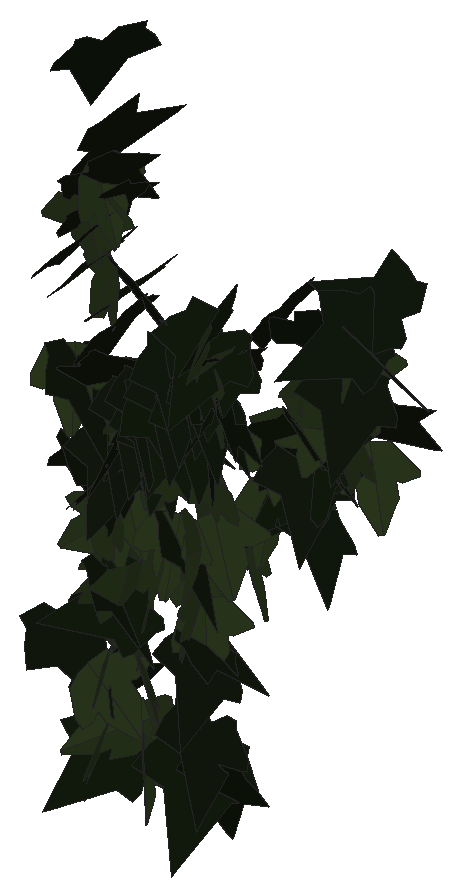
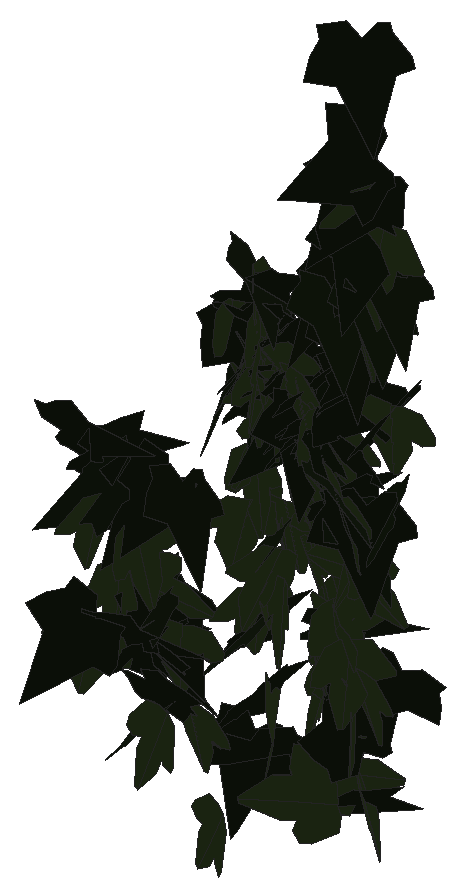
# SketchUp Ruby script. Lengths in inches.
U = 1.inch
M = Sketchup.active_model
def pt(a) = Geom::Point3d.new(a.map { |v| v * U })
def face(e, loops, mat)
  f = e.add_face(loops[0].map { |a| pt(a) })
  loops[1..].each { |l| e.add_face(l.map { |a| pt(a) }).erase! }
  f.material = f.back_material = mat if mat
  f
end
# faces: each face lists its corners as indices into pts; further lists are holes
def faces(e, pts, list, mat = nil) = list.each { |f| face(e, (f[0].is_a?(Array) ? f : [f]).map { |l| l.map { |i| pts[i] } }, mat) }
# xy, xz, yz: faces in a plane at the given z, y or x. An outline is a flat list of corners, or four numbers for a rectangle; further outlines are holes
def ring(l) = l.size == 4 ? [[l[0], l[1]], [l[2], l[1]], [l[2], l[3]], [l[0], l[3]]] : l.each_slice(2).to_a
def flat(e, list, mat, &to3) = list.each { |f| face(e, (f[0].is_a?(Array) ? f : [f]).map { |l| ring(l).map { |u, v| to3.(u, v) } }, mat) }
def xy(e, z, list, mat = nil) = flat(e, list, mat) { |x, y| [x, y, z] }
def xz(e, y, list, mat = nil) = flat(e, list, mat) { |x, z| [x, y, z] }
def yz(e, x, list, mat = nil) = flat(e, list, mat) { |y, z| [x, y, z] }
def lines(e, pts, list) = list.each { |a, b| e.add_line(pt(pts[a]), pt(pts[b])) }
# prism: a flat outline (further loops are holes) pulled along v
def prism(e, loops, v, mat = nil)
  f = face(e, loops, mat); d = Geom::Vector3d.new(v.map { |x| x * U })
  f.pushpull(f.normal.samedirection?(d) ? d.length : -d.length)
end
def box(e, o, s, mat = nil) = prism(e, [[o, [o[0] + s[0], o[1], o[2]], [o[0] + s[0], o[1] + s[1], o[2]], [o[0], o[1] + s[1], o[2]]]], [0, 0, s[2]], mat)
def at(x, y, z, deg = 0) = Geom::Transformation.translation(pt([x, y, z])) * Geom::Transformation.rotation(ORIGIN, Z_AXIS, deg.degrees)
def axes(o, x, y, z) = Geom::Transformation.new([*x, 0, *y, 0, *z, 0, *pt(o).to_a, 1])
def part(name) = M.definitions.add(name)
# library, detail: a bought-in or finely detailed component or shape, given as its bounding box
def library(name, o, s) = part(name).tap { |d| box(d.entities, o, s) }
def detail(e, o, s) = box(e.add_group.entities, o, s)
def put(e, d, t, mat = nil) = e.add_instance(d, t).tap { |i| i.material = mat if mat }
def group(e, t, mat = nil) = e.add_group.tap { |g| g.transformation = t; g.material = mat if mat }.entities
root = M.entities
M.materials.add("efeu1").color = [18, 25, 13]
M.materials.add("efeu2").color = [43, 57, 29]
c1 = part("ivyleaf_9")
p = [[1.54,2.16,1.25],[1.36,2.04,1.19],[-0.21,0.99,0.68],[-0.71,1.11,0.82],[-0.85,0.86,0.67],[-0.8,0.17,0.21],
  [-0.9,-0.01,0.1],[-0.67,-0.16,-0.02],[-0.08,-0.08,-0.05],[-0.03,-0.6,-0.4],[0.65,-0.88,-0.66],[0.83,-0.6,-0.49],
  [1.29,-0.42,-0.43],[1.8125,-0.07,-0.26],[1.21,0.44,0.15]]
faces(c1.entities,p,[[0,1,2,3,4,5,6,7,8,9,10,11,12,13,14]],"efeu1")
c2 = part("ivyleaf_10")
p = [[0,0.5,-0.03],[-0.0625,2.02,-0.43],[-0.19,2.01,-0.46],[-0.54,1.05,-0.29],[-0.52,0.625,-0.18],[-0.83,0.76,-0.28],
  [-1.16,0.64,-0.33],[-1.15,0.33,-0.24],[-0.77,-0.39,0.02],[-0.3,-0.51,0.16],[0.04,-0.48,0.23],[-0.02,2.01,-0.4375],
  [-0.06,2.01,-0.43],[0.04,-0.49,0.23],[0.67,-0.49,0.14],[1.38,0.36,-0.2],[1.375,0.51,-0.24],[0.81,0.65,-0.19],
  [0.62,0.59,-0.15],[0.6,1.09,-0.28],[0.5,1.23,-0.31]]
faces(c2.entities,p,[[0,1,2,3,4,5,6,7,8,9,10],[11,12,0,13,14,15,16,17,18,19,20]],"efeu2")
put(root,c1,axes([535.11,135.38,196.85],[-0.09236,0.78895,0.04557],[-0.11225,0.03231,-0.78703],[-0.78225,-0.09779,0.10755]))
put(root,c1,axes([534.95,136.32,191.54],[0.27954,0.64457,-0.3045],[-0.13089,-0.27511,-0.70251],[-0.70076,0.30851,0.00975]))
put(root,c2,axes([534.64,141.72,186.61],[-0.55689,0.38935,-0.31691],[0.20976,-0.24955,-0.67519],[-0.4561,-0.59015,0.07643]))
put(root,c2,axes([534.65,135.8125,193.64],[0.75631,0.15159,0.10744],[0.10414,0.02707,-0.77133],[-0.15387,0.76342,0.00602]))
put(root,c1,axes([534.5,136.11,191.47],[0.57095,-0.50219,-0.11891],[-0.09775,0.06889,-0.76028],[0.50674,0.57912,-0.01267]))
put(root,c1,axes([535.26,135.63,196.22],[-0.0272,0.76113,0.20937],[-0.17444,0.19852,-0.74435],[-0.76988,-0.07187,0.16126]))
put(root,c2,axes([534.9,136.51,187.58],[0.67301,-0.30708,-0.03386],[-0.02998,0.01585,-0.73976],[0.30748,0.67368,0.00197]))
put(root,c2,axes([535.29,136.23,189.9375],[0.50596,0.01664,-0.55127],[-0.54853,0.09291,-0.50064],[0.0573,0.74246,0.075]))
put(root,c1,axes([534.57,135.6875,187.55],[-0.23146,-0.33322,-0.67897],[0.48601,0.47853,-0.40053],[0.57951,-0.5344,0.06472]))
put(root,c2,axes([535.0625,136.77,188.2],[-0.38763,-0.62413,-0.09349],[0.07627,0.06258,-0.73403],[0.62646,-0.3938,0.03152]))
put(root,c1,axes([534.72,135.92,193.66],[0.26543,-0.73695,-0.07388],[-0.01248,0.07402,-0.78318],[0.74054,0.26539,0.01328]))
put(root,c2,axes([535.13,135.7,197.53],[-0.75386,-0.22402,-0.07222],[0.0647,0.03576,-0.78628],[0.22631,-0.75646,-0.01578]))
put(root,c2,axes([535.51,135.96,190.48],[-0.51529,0.27531,0.48439],[-0.49254,0.08332,-0.57132],[-0.26044,-0.70229,0.1221]))
put(root,c1,axes([535.52,135.98,191.26],[-0.24376,0.71357,-0.08922],[-0.05412,-0.11214,-0.74903],[-0.71708,-0.2341,0.08686]))
put(root,c2,axes([535.22,136.07,184.8],[0.39934,-0.69556,-0.0429],[-0.02049,0.0377,-0.80204],[0.69658,0.39986,0.001]))
put(root,c2,axes([535.46,135.76,190.25],[-0.10227,0.22738,0.8121],[-0.4068,0.70329,-0.24814],[-0.73873,-0.41876,0.02422]))
put(root,c2,axes([535.38,136.75,189.04],[-0.25145,-0.69267,0.08762],[-0.04017,-0.07862,-0.73682],[0.69703,-0.25441,-0.01086]))
put(root,c1,axes([535.39,135.7,197.68],[0.23465,0.75171,0.08399],[-0.00719,0.09015,-0.78676],[-0.75635,0.23235,0.03353]))
put(root,c1,axes([535.5,136.4375,184.48],[-0.5673,-0.42169,0.28675],[-0.11799,-0.30876,-0.68748],[0.49611,-0.55563,0.1644]))
put(root,c2,axes([535.46,136.04,186.88],[0.28678,-0.65018,-0.41383],[-0.05057,0.42473,-0.70234],[0.76905,0.27038,0.10814]))
put(root,c2,axes([535.55,135.875,196],[0.5749,-0.3788,-0.38537],[-0.23953,0.32573,-0.67752],[0.48438,0.61067,0.12235]))
put(root,c2,axes([535.7,136.47,185.09],[-0.16062,-0.08458,0.73787],[-0.27876,-0.69287,-0.1401],[0.68841,-0.3003,0.11543]))
put(root,c1,axes([535.17,136.24,185.82],[0.48747,0.54379,0.24016],[-0.16774,-0.17213,0.73024],[0.5703,-0.51544,0.0095]))
put(root,c2,axes([535.01,136.76,190.38],[0.15973,-0.00641,0.72515],[0.72497,-0.01607,-0.15983],[0.01707,0.74236,0.0028]))
put(root,c1,axes([536.12,136.18,192.07],[-0.32542,0.62202,0.30151],[-0.26774,0.19381,-0.68882],[-0.63728,-0.39905,0.13543]))
put(root,c1,axes([535.82,135.4,201.85],[0.14151,0.74554,-0.29304],[-0.04633,-0.28946,-0.75881],[-0.79972,0.14869,-0.00789]))
put(root,c2,axes([535.125,136.55,191.125],[0.46745,-0.14604,-0.5731],[0.56414,-0.10918,0.48796],[-0.17753,-0.73146,0.04158]))
put(root,c2,axes([535.53,135.69,198.4],[0.05691,0.7923,0.09417],[-0.00039,0.09444,-0.79431],[-0.79788,0.05646,0.00711]))
put(root,c1,axes([535.99,135.71,190.74],[0.05917,0.18429,0.8318],[-0.21698,0.80957,-0.16393],[-0.82388,-0.19997,0.10292]))
put(root,c1,axes([535.62,136.4,191.68],[-0.30342,-0.68109,0.14956],[-0.00635,-0.1604,-0.74334],[0.69729,-0.29783,0.05831]))
put(root,c1,axes([535.57,135.33,198.69],[0.50806,0.59704,0.19702],[0.10908,0.16576,-0.7836],[-0.61917,0.5191,0.02362]))
put(root,c1,axes([535.38,135.39,193.95],[0.69662,0.30861,0.19682],[0.16615,0.11043,-0.76122],[-0.32614,0.71542,0.0326]))
put(root,c1,axes([535.55,135.42,199.2],[0.32111,0.40499,0.72526],[0.38216,0.61837,-0.5145],[-0.73755,0.49673,0.04917]))
put(root,c1,axes([536.25,136.17,188.27],[-0.5468,-0.12696,0.51847],[-0.4596,-0.26548,-0.54973],[0.27146,-0.70521,0.11361]))
put(root,c1,axes([536.16,135.8125,195.85],[-0.01524,0.76874,0.18462],[-0.18849,0.17579,-0.74756],[-0.7678,-0.05841,0.17985]))
put(root,c1,axes([535.48,135.97,188.87],[0.45083,-0.60687,-0.11641],[-0.05317,0.10547,-0.75574],[0.61565,0.45351,0.01998]))
put(root,c2,axes([535.4,136.74,188.6875],[0.52779,-0.1297,0.50611],[0.5153,0.0105,-0.53469],[0.08622,0.73117,0.09746]))
put(root,c2,axes([535.76,140.98,188.5],[0.74009,-0.16077,0.0819],[0.07781,-0.0276,-0.75728],[0.16279,0.74409,-0.01039]))
put(root,c1,axes([536.16,135.31,195.25],[-0.07575,0.78324,0.03306],[-0.00511,0.03272,-0.78689],[-0.78392,-0.07589,0.00193]))
put(root,c2,axes([535.66,135.46,186.58],[0.27132,0.61797,0.40989],[0.16811,0.37385,-0.6749],[-0.72224,0.31916,-0.00311]))
put(root,c2,axes([535.88,142.05,188.6],[-0.68069,0.31597,-0.11703],[0.10346,-0.05507,-0.75042],[-0.32067,-0.68848,0.00631]))
put(root,c2,axes([536.05,135.77,188.99],[-0.14466,-0.72566,0.0885],[-0.00606,-0.08902,-0.73985],[0.73101,-0.14434,0.01138]))
put(root,c2,axes([535.85,136.21,190.93],[-0.72002,-0.19323,-0.19757],[0.25425,-0.24714,-0.68489],[0.10829,-0.70454,0.29443]))
put(root,c2,axes([536.07,136.04,192.69],[-0.72768,-0.2288,0.03372],[0.03191,-0.20961,-0.73352],[0.22906,-0.69766,0.20932]))
put(root,c1,axes([535.9375,136.1875,192.74],[-0.57233,-0.2298,-0.46523],[0.4506,0.12338,-0.61526],[0.25732,-0.72717,0.04263]))
put(root,c2,axes([536.2,136.29,193.06],[-0.0617,-0.7643,-0.04049],[-0.00636,0.04113,-0.76673],[0.76535,-0.06127,-0.00964]))
put(root,c2,axes([536.01,136.67,188.05],[0.46257,-0.55914,0.17539],[0.14466,-0.10758,-0.72448],[0.56787,0.48287,0.04168]))
put(root,c1,axes([536.42,140.53,193.4375],[-0.14999,0.74483,-0.05611],[0.01282,-0.05466,-0.75978],[-0.74683,-0.15052,-0.00177]))
put(root,c1,axes([536.29,136.02,192.96],[-0.39585,0.3905,-0.52634],[0.31455,-0.42625,-0.55281],[-0.57496,-0.50204,0.05995]))
put(root,c2,axes([535.99,136.4,192.09],[0.62776,-0.33463,0.27332],[0.30094,-0.00728,-0.70011],[0.31003,0.68465,0.12615]))
put(root,c1,axes([536.57,141.46,189.16],[-0.76077,-0.0903,-0.02056],[0.02036,0.00287,-0.76611],[0.09035,-0.76105,-0.00045]))
put(root,c2,axes([536.36,136.05,186.875],[-0.53735,0.53884,0.05885],[-0.04078,0.04244,-0.76099],[-0.54051,-0.5389,-0.00109]))
put(root,c2,axes([535.72,136.93,184.64],[0.1309,-0.02135,0.88207],[0.7811,0.41754,-0.10581],[-0.41036,0.78794,0.07997]))
put(root,c2,axes([536.24,140.76,190.07],[0.6887,0.26199,0.09397],[0.0809,0.05154,-0.7366],[-0.26631,0.69317,0.01925]))
put(root,c1,axes([536.3125,135.55,196.36],[0.71728,-0.03176,-0.32894],[-0.32544,0.06873,-0.71629],[0.05743,0.78611,0.04933]))
put(root,c1,axes([536.33,136.25,193.23],[-0.19239,-0.74429,0.01304],[-0.00296,-0.0127,-0.76875],[0.7444,-0.19241,0.00031]))
put(root,c2,axes([536.74,135.9375,189.71],[0.45253,-0.41829,-0.4238],[-0.30326,0.2962,-0.61616],[0.51245,0.54466,0.00961]))
put(root,c2,axes([536.34,136.23,184.74],[-0.1883,0.54769,-0.47254],[0.15472,-0.44649,-0.57916],[-0.70663,-0.24371,-0.00089]))
put(root,c1,axes([536.74,135.97,192.97],[0.14289,0.74984,-0.03204],[-0.0069,-0.0313,-0.76334],[-0.7505,0.14305,0.00091]))
put(root,c1,axes([536.94,140.62,190.59],[0.22843,0.41205,-0.61528],[-0.38947,-0.48078,-0.46658],[-0.62981,0.44677,0.06537]))
put(root,c2,axes([536.66,136.33,191.65],[0.37013,-0.6507,-0.01195],[-0.00372,0.01163,-0.7486],[0.6508,0.37014,0.00252]))
put(root,c2,axes([537.28,140.58,190.88],[0.17253,-0.04008,-0.75614],[-0.74934,0.10242,-0.17641],[0.10882,0.76878,-0.01592]))
put(root,c1,axes([537.09,140.95,189.64],[-0.76577,0.02598,0.00332],[-0.00283,0.01447,-0.76608],[-0.02604,-0.76564,-0.01436]))
put(root,c2,axes([536.74,136.23,193.67],[0.42276,-0.64464,0.02235],[0.06418,0.01545,-0.76839],[0.64183,0.42307,0.06211]))
put(root,c2,axes([536.37,136.12,192.9375],[0.60601,0.03605,0.48638],[0.48562,0.02735,-0.60708],[-0.04523,0.77658,-0.0012]))
put(root,c2,axes([536.99,136.66,188.92],[-0.58959,0.42707,0.17582],[-0.20883,0.00778,-0.7192],[-0.41193,-0.6152,0.11296]))
put(root,c1,axes([536.58,136.3125,192.82],[0.11383,-0.75777,-0.01867],[0.00266,0.01928,-0.76625],[0.75799,0.11373,0.00549]))
put(root,c1,axes([536.73,136.23,192.94],[-0.0844,-0.76088,0.08691],[0.00819,-0.08833,-0.76534],[0.76578,-0.08292,0.01777]))
put(root,c2,axes([536.9375,136.13,193.15],[0.68141,-0.32662,-0.07074],[-0.06354,0.0311,-0.75564],[0.3281,0.68436,0.00058]))
put(root,c1,axes([536.72,136.11,193.625],[-0.05822,-0.773,0.08201],[0.00858,-0.08287,-0.77505],[0.77729,-0.05698,0.0147]))
put(root,c1,axes([536.625,141.52,188.14],[0.09204,-0.73,0.19546],[0.13901,-0.17719,-0.72723],[0.74282,0.12361,0.11187]))
put(root,c1,axes([537.59,141.64,190.12],[-0.58265,0.13379,0.48618],[-0.49948,-0.05123,-0.5845],[-0.06916,-0.75711,0.12546]))
put(root,c1,axes([536.71,136.1,193.1],[0.76092,0.06318,0.00846],[0.00301,0.0657,-0.76075],[-0.06367,0.75813,0.06522]))
put(root,c1,axes([536.9,141,189.76],[-0.18793,-0.74405,-0.04972],[0.02212,0.04569,-0.76735],[0.74538,-0.18895,0.01024]))
put(root,c1,axes([536.73,140.68,190.82],[0.68302,-0.33314,-0.14426],[-0.11878,0.08537,-0.75954],[0.34305,0.69284,0.02423]))
put(root,c2,axes([537.18,136.03,192.69],[0.09995,-0.7706,-0.10232],[0.04342,0.10853,-0.775],[0.77615,0.09316,0.05653]))
put(root,c2,axes([537.39,136.29,194.2],[0.65017,-0.00814,-0.4095],[-0.40956,-0.00691,-0.65014],[0.00321,0.76834,-0.01019]))
put(root,c2,axes([537.26,140.95,192.1],[-0.12945,-0.76481,0.07929],[-0.0065,-0.07931,-0.77566],[0.76888,-0.12944,0.00679]))
put(root,c1,axes([536.97,140.45,193.33],[0.67626,0.36695,-0.01396],[-0.01269,-0.00588,-0.7694],[-0.36699,0.67638,0.00089]))
put(root,c2,axes([537.16,136.18,193.88],[0.72656,-0.25353,-0.00901],[-0.00723,0.00663,-0.76951],[0.25358,0.72658,0.00388]))
put(root,c1,axes([537.09,135.68,193.54],[0.72432,0.12056,-0.23583],[-0.24402,0.03676,-0.73068],[-0.10298,0.76086,0.07267]))
put(root,c2,axes([537.27,136.53,189.54],[0.16018,0.65025,0.34878],[-0.01267,0.35927,-0.66399],[-0.73777,0.13501,0.08713]))
put(root,c1,axes([537.33,136.09,193.62],[-0.4749,-0.59863,-0.09803],[0.12064,0.02881,-0.76033],[0.59448,-0.48405,0.07598]))
put(root,c2,axes([537.28,135.93,190.47],[0.74941,0.05873,0.00738],[0.00672,0.00867,-0.75167],[-0.05881,0.7494,0.00812]))
put(root,c1,axes([537.15,135.82,193.76],[0.04536,-0.74269,-0.27181],[-0.01618,0.27133,-0.74407],[0.7907,0.04816,0.00037]))
put(root,c1,axes([537.39,136.16,194.03],[-0.22142,-0.74001,-0.0517],[0.02059,0.0478,-0.7724],[0.74152,-0.22229,0.00601]))
put(root,c2,axes([537.6,136.32,193.84],[-0.2838,-0.70143,-0.11364],[0.06995,0.0942,-0.7561],[0.70712,-0.29083,0.02919]))
put(root,c1,axes([537.2,136.24,190.28],[0.40071,-0.65686,0.0679],[0.03005,-0.0612,-0.76941],[0.65967,0.40179,-0.00619]))
put(root,c2,axes([537.28,136.61,185.6],[-0.013,0.05909,-0.90042],[0.31522,-0.84349,-0.0599],[-0.84551,-0.31538,-0.00849]))
put(root,c2,axes([537.91,136.38,191.625],[-0.68226,0.14655,0.28738],[-0.29377,-0.00444,-0.69514],[-0.1333,-0.7403,0.06106]))
put(root,c2,axes([537.68,136.29,194.18],[0.17304,-0.63867,-0.38998],[0.04045,0.40767,-0.64969],[0.74722,0.12583,0.12548]))
put(root,c2,axes([537.53,136.16,193.6],[0.3607,0.66502,0.02328],[0.01262,0.01964,-0.75654],[-0.66531,0.36091,-0.00173]))
put(root,c1,axes([537.47,135.99,194.62],[-0.05334,-0.78164,-0.01296],[-0.00311,0.0132,-0.78344],[0.78174,-0.05328,-0.004]))
put(root,c2,axes([537.77,136.22,194.78],[0.06263,-0.76021,-0.12697],[0.02667,0.12945,-0.7619],[0.77028,0.05733,0.0367]))
put(root,c1,axes([537.55,142.13,190.56],[0.60091,0.46244,0.13789],[0.0835,0.11725,-0.75712],[-0.47528,0.60527,0.04132]))
put(root,c2,axes([537.99,140.84,190.75],[-0.69259,0.24129,0.24295],[-0.2369,0.05814,-0.73309],[-0.24723,-0.73166,0.02186]))
put(root,c2,axes([537.69,136.22,188.89],[0.26581,-0.60205,0.36787],[0.19738,-0.31396,-0.65645],[0.67738,0.32774,0.04693]))
put(root,c1,axes([537.81,136.48,185.11],[-0.614,-0.64025,-0.18777],[0.1304,0.1351,-0.88708],[0.65435,-0.6277,0.00059]))
put(root,c1,axes([537.62,136.39,193.51],[-0.03833,-0.76074,-0.01951],[0.00108,0.01948,-0.76171],[0.76099,-0.03835,0.0001]))
put(root,c2,axes([537.73,135.68,192.3125],[-0.30352,-0.53722,-0.50659],[0.32692,0.39334,-0.613],[0.66209,-0.4405,0.07044]))
put(root,c2,axes([538.23,135.36,190.59],[0.29282,-0.40858,-0.62654],[-0.37439,0.50243,-0.50262],[0.64755,0.47525,-0.00728]))
put(root,c1,axes([538.34,135.76,193.93],[-0.58188,0.49491,0.0287],[-0.02332,0.01687,-0.76388],[-0.49519,-0.58234,0.00226]))
put(root,c1,axes([537.61,136.18,188.19],[0.60717,-0.33842,-0.3488],[-0.16364,0.38321,-0.65667],[0.45762,0.58606,0.22797]))
put(root,c2,axes([537.86,136.26,188.47],[0.31654,0.68252,-0.01434],[-0.02429,-0.00453,-0.75208],[-0.68224,0.31684,0.02012]))
put(root,c1,axes([538.49,135.48,195.62],[-0.18347,0.6337,0.41989],[-0.1873,0.38094,-0.65676],[-0.73675,-0.25465,0.06241]))
put(root,c1,axes([538.46,136.09,194.8125],[-0.10666,0.65874,-0.37637],[-0.11157,-0.38956,-0.6502],[-0.75043,-0.03572,0.15016]))
put(root,c2,axes([537.89,141.69,189.82],[0.67402,0.30834,0.20555],[0.18954,0.07976,-0.74117],[-0.31843,0.70013,-0.00609]))
put(root,c1,axes([538.01,136.17,187.68],[-0.14507,-0.74048,0.20974],[-0.02648,-0.2085,-0.75443],[0.76915,-0.14684,0.01359]))
put(root,c1,axes([538.19,136.01,184.98],[0.59468,0.33357,-0.33422],[-0.27874,-0.18585,-0.68146],[-0.38115,0.65636,-0.0231]))
put(root,c2,axes([538,136.46,190.48],[0.48289,0.5634,0.16834],[0.07604,0.15616,-0.7408],[-0.58308,0.48697,0.0428]))
put(root,c1,axes([537.9,136.22,194.2],[0.41669,-0.60943,-0.21998],[-0.12721,0.17949,-0.73825],[0.6353,0.43566,-0.00355]))
put(root,c2,axes([538.26,135.76,195.47],[0.31365,-0.70807,-0.08746],[0.05992,0.12134,-0.76751],[0.71093,0.30216,0.10327]))
put(root,c2,axes([538.06,136.01,194.45],[-0.47285,0.40582,-0.44301],[0.28161,-0.34828,-0.61962],[-0.53069,-0.54639,0.06592]))
put(root,c1,axes([538.06,136.14,186],[-0.06405,-0.7929,0.15389],[0.01984,-0.15587,-0.79485],[0.80746,-0.05907,0.03174]))
put(root,c1,axes([537.87,136.32,193.07],[0.10503,-0.04732,-0.75654],[0.70991,-0.26163,0.11492],[-0.26575,-0.71759,0.00799]))
put(root,c1,axes([538.35,136.09,195.43],[-0.45886,-0.61975,0.07357],[-0.05381,-0.05168,-0.77103],[0.62177,-0.46184,-0.01244]))
put(root,c1,axes([537.99,136.17,194.06],[0.11786,-0.74625,0.12209],[0.05575,-0.11465,-0.75461],[0.75412,0.12511,0.03671]))
put(root,c1,axes([538.27,136.18,194.96],[-0.53174,-0.49871,-0.25576],[0.20248,0.1578,-0.72868],[0.52261,-0.56856,0.0221]))
put(root,c2,axes([538.31,140.99,192.5],[0.08993,0.74499,0.07381],[-0.03421,0.07835,-0.74915],[-0.74785,0.086,0.04314]))
put(root,c2,axes([538.47,136.22,194.83],[-0.08067,-0.76041,-0.00077],[-0.00045,0.00083,-0.76468],[0.76041,-0.08067,-0.00054]))
put(root,c1,axes([538.68,140.67,193.56],[-0.43115,-0.40163,0.52611],[-0.38804,-0.35528,-0.58922],[0.53621,-0.58005,-0.00338]))
put(root,c1,axes([537.94,140.92,193.1875],[0.73603,-0.25988,0.08859],[0.1007,0.01971,-0.77885],[0.25543,0.74108,0.05178]))
put(root,c1,axes([538.4,136.18,193.92],[0.497,-0.25128,-0.5307],[-0.46399,0.25803,-0.55671],[0.35985,0.67976,0.01515]))
put(root,c1,axes([539.14,141.02,194.02],[-0.38212,0.20612,0.62733],[-0.60085,0.19209,-0.4291],[-0.27388,-0.70899,0.06612]))
put(root,c1,axes([538.41,140.62,192.33],[-0.26462,-0.7383,0.0523],[0.02659,-0.06499,-0.78289],[0.73967,-0.26179,0.04686]))
